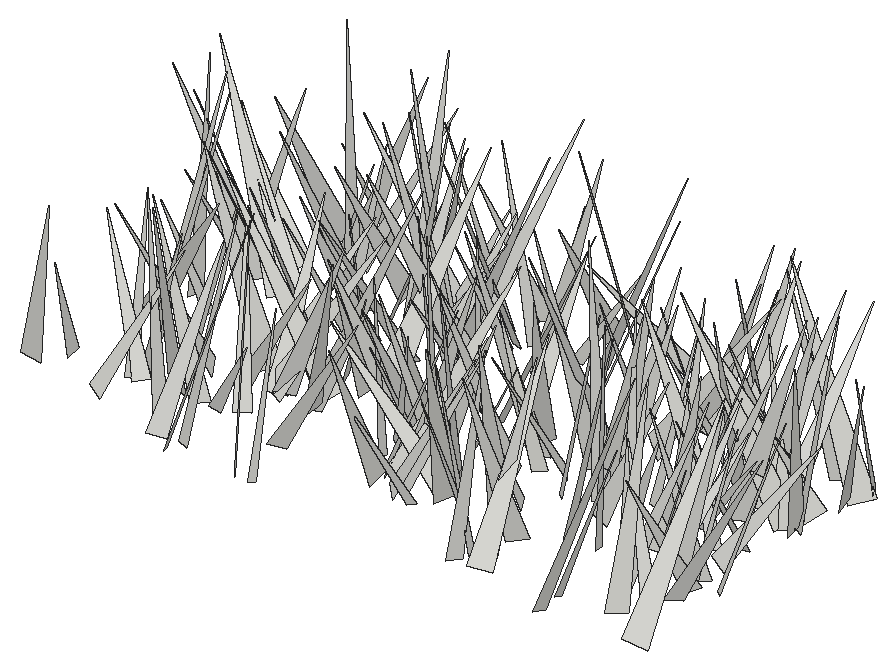
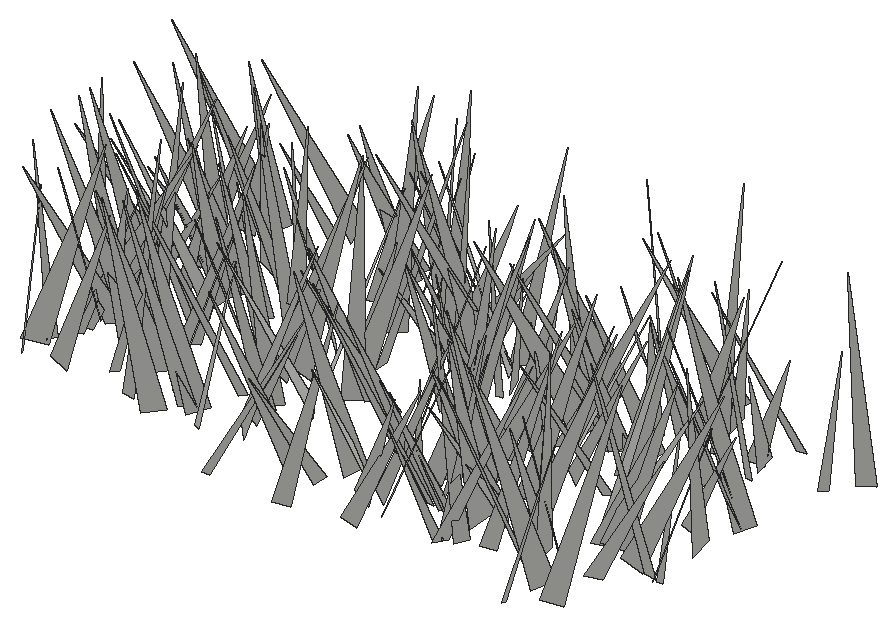
# SketchUp Ruby script. Lengths in inches.
U = 1.inch
M = Sketchup.active_model
def pt(a) = Geom::Point3d.new(a.map { |v| v * U })
def face(e, loops, mat)
  f = e.add_face(loops[0].map { |a| pt(a) })
  loops[1..].each { |l| e.add_face(l.map { |a| pt(a) }).erase! }
  f.material = f.back_material = mat if mat
  f
end
# faces: each face lists its corners as indices into pts; further lists are holes
def faces(e, pts, list, mat = nil) = list.each { |f| face(e, (f[0].is_a?(Array) ? f : [f]).map { |l| l.map { |i| pts[i] } }, mat) }
# xy, xz, yz: faces in a plane at the given z, y or x. An outline is a flat list of corners, or four numbers for a rectangle; further outlines are holes
def ring(l) = l.size == 4 ? [[l[0], l[1]], [l[2], l[1]], [l[2], l[3]], [l[0], l[3]]] : l.each_slice(2).to_a
def flat(e, list, mat, &to3) = list.each { |f| face(e, (f[0].is_a?(Array) ? f : [f]).map { |l| ring(l).map { |u, v| to3.(u, v) } }, mat) }
def xy(e, z, list, mat = nil) = flat(e, list, mat) { |x, y| [x, y, z] }
def xz(e, y, list, mat = nil) = flat(e, list, mat) { |x, z| [x, y, z] }
def yz(e, x, list, mat = nil) = flat(e, list, mat) { |y, z| [x, y, z] }
def lines(e, pts, list) = list.each { |a, b| e.add_line(pt(pts[a]), pt(pts[b])) }
# prism: a flat outline (further loops are holes) pulled along v
def prism(e, loops, v, mat = nil)
  f = face(e, loops, mat); d = Geom::Vector3d.new(v.map { |x| x * U })
  f.pushpull(f.normal.samedirection?(d) ? d.length : -d.length)
end
def box(e, o, s, mat = nil) = prism(e, [[o, [o[0] + s[0], o[1], o[2]], [o[0] + s[0], o[1] + s[1], o[2]], [o[0], o[1] + s[1], o[2]]]], [0, 0, s[2]], mat)
def at(x, y, z, deg = 0) = Geom::Transformation.translation(pt([x, y, z])) * Geom::Transformation.rotation(ORIGIN, Z_AXIS, deg.degrees)
def axes(o, x, y, z) = Geom::Transformation.new([*x, 0, *y, 0, *z, 0, *pt(o).to_a, 1])
def part(name) = M.definitions.add(name)
# library, detail: a bought-in or finely detailed component or shape, given as its bounding box
def library(name, o, s) = part(name).tap { |d| box(d.entities, o, s) }
def detail(e, o, s) = box(e.add_group.entities, o, s)
def put(e, d, t, mat = nil) = e.add_instance(d, t).tap { |i| i.material = mat if mat }
def group(e, t, mat = nil) = e.add_group.tap { |g| g.transformation = t; g.material = mat if mat }.entities
root = M.entities
c1 = part("fur_instance\#9")
p = [[0.8125,0,1.79],[0.67,-0.02,1.48],[0,-0.11,0],[0,0.11,0]]
faces(c1.entities,p,[[0,1,2,3]])
put(root,c1,axes([541.47,408.85,-21.66],[7.3603,1.92647,1.4977],[1.22652,-7.03518,3.02165],[-2.10951,2.63124,6.98247]))
put(root,c1,axes([533.68,410.5,-21.66],[-6.0255,1.4926,2.28597],[0.94971,6.33899,-1.63567],[2.5596,1.16168,5.98825]))
put(root,c1,axes([524.07,415.33,-21.66],[6.25747,-1.85529,1.59771],[-1.00282,-5.94215,-2.97253],[-2.23363,-2.52972,5.81052]))
put(root,c1,axes([516.98,410.62,-21.66],[5.31118,5.11176,2.74997],[4.78098,-5.96627,1.85658],[-3.29161,-0.41778,7.13385]))
put(root,c1,axes([548.43,409.16,-21.66],[-1.16046,8.00046,0.20395],[7.87345,1.17823,-1.41992],[1.43448,0.00519,7.95851]))
put(root,c1,axes([535.15,414.7,-21.66],[2.99002,-5.93259,1.12286],[-5.76165,-3.17812,-1.449],[-1.8055,0.31717,6.48354]))
put(root,c1,axes([531.17,414.73,-21.66],[-4.0085,-3.44331,0.94309],[-3.06456,4.04605,1.74695],[1.83147,-0.76613,4.98725]))
put(root,c1,axes([498.86,413.9375,-21.66],[1.26894,-6.32164,1.3833],[-6.3592,-0.957,1.46001],[1.19887,1.6149,6.28026]))
put(root,c1,axes([534.1,411.68,-21.66],[-5.43034,-1.89464,0.64767],[-1.9986,5.01546,-2.08529],[-0.12137,2.18018,5.36002]))
put(root,c1,axes([541.21,410.91,-21.66],[4.47299,1.54799,0.88013],[1.09405,-4.26651,1.94385],[-1.40498,1.60599,4.31572]))
put(root,c1,axes([518.46,410.37,-21.66],[1.86893,4.92203,0.04113],[4.36091,-1.67616,2.42774],[-2.28266,0.8277,4.67176]))
put(root,c1,axes([528.74,416.03,-21.66],[6.44625,-4.17663,0.34492],[-3.99481,-6.31514,-1.81045],[-1.26676,-1.33867,7.46462]))
put(root,c1,axes([527.57,414.14,-21.66],[-0.38653,-3.78857,0.47263],[-3.40937,0.1287,-1.7566],[-1.71837,0.59684,3.37891]))
put(root,c1,axes([545.21,411.5,-21.66],[-6.19625,3.45387,1.64148],[3.0912,6.3638,-1.72156],[2.25127,0.76815,6.88178]))
put(root,c1,axes([535.02,411.81,-21.66],[5.43487,-1.88004,3.06705],[-2.9758,-5.47185,1.91904],[-2.02138,3.00059,5.42123]))
put(root,c1,axes([512.02,410.2,-21.66],[6.2923,4.31715,0.79405],[3.75537,-6.01297,2.93303],[-2.27277,2.01685,7.04472]))
put(root,c1,axes([507.96,416.44,-21.66],[-1.88375,-7.99896,1.23534],[-7.80751,2.13018,1.88761],[2.13359,0.73274,7.99805]))
put(root,c1,axes([546.625,412.86,-21.66],[-1.63602,4.97918,0.62205],[4.87533,1.42244,1.43652],[-1.18757,-1.0199,5.04036]))
put(root,c1,axes([547.03,416.39,-21.66],[2.87484,-4.36178,0.57915],[-3.91954,-2.85297,-2.03053],[-1.99945,-0.67874,4.81319]))
put(root,c1,axes([512.45,411.35,-21.66],[3.92721,6.27569,0.86047],[6.07775,-4.01843,1.56873],[-1.78486,0.12492,7.23508]))
put(root,c1,axes([535.59,410.5,-21.66],[-4.59589,5.78444,0.11594],[5.4804,4.40003,-2.28044],[1.8543,1.33244,7.02721]))
put(root,c1,axes([510.55,411.1875,-21.66],[-4.56425,4.1816,0.8559],[3.58274,4.43445,-2.55936],[2.31998,1.37862,5.63629]))
put(root,c1,axes([504.38,413.08,-21.66],[2.28513,5.39499,0.34939],[5.12885,-2.04337,-1.99232],[1.70965,-1.08097,5.50984]))
put(root,c1,axes([500.49,415.91,-21.66],[4.01864,-1.00258,0.99057],[-0.63294,-3.95809,-1.43832],[-1.25928,-1.21004,3.88405]))
put(root,c1,axes([532.2,416.79,-21.66],[6.58115,-3.41587,1.26301],[-3.10443,-6.62563,-1.74311],[-1.90417,-1.00387,7.20703]))
put(root,c1,axes([516.94,414.61,-21.66],[4.74645,-3.63152,0.20608],[-3.44873,-4.38539,2.15263],[1.15614,1.82746,5.57521]))
put(root,c1,axes([509.33,413.1,-21.66],[-6.71,0.21588,0.88951],[-0.0468,6.49159,-1.92847],[0.91413,1.91692,6.43053]))
put(root,c1,axes([543.35,414.43,-21.66],[2.52048,5.79703,1.2985],[5.75928,-2.03853,-2.07834],[1.45681,-1.97061,5.96983]))
put(root,c1,axes([525.625,414.61,-21.66],[4.10268,4.53992,0.30052],[4.35228,-3.79801,-2.04106],[1.3262,-1.58032,5.76861]))
put(root,c1,axes([511.33,415.82,-21.66],[1.52564,-3.34819,0.07276],[-3.07421,-1.36842,1.48995],[1.32851,0.67846,3.36423]))
put(root,c1,axes([546.86,414.81,-21.66],[5.8068,-2.41673,0.19711],[-2.36119,-5.5195,1.88633],[0.55156,1.81463,6.0001]))
put(root,c1,axes([528.11,416.6,-21.66],[-5.02457,3.67244,0.21301],[3.24783,4.25941,3.17608],[-1.72736,-2.67378,5.35216]))
put(root,c1,axes([525.98,415.22,-21.66],[3.52755,5.08967,0.59914],[4.90233,-3.13928,-2.19532],[1.49362,-1.71683,5.79042]))
put(root,c1,axes([543.72,416.86,-21.66],[4.89387,1.35478,0.49174],[1.44124,-4.60961,-1.64362],[-0.00784,-1.71558,4.80457]))
put(root,c1,axes([528.08,417.97,-21.66],[-6.05203,-3.65216,2.90127],[-3.20675,6.70926,1.75646],[3.38709,-0.1736,6.84691]))
put(root,c1,axes([532.67,418.22,-21.66],[-3.8372,-2.33717,0.79383],[-2.01321,3.81242,1.493],[1.42812,-0.90538,4.23762]))
put(root,c1,axes([523.78,416.45,-21.66],[5.98281,3.47845,0.55141],[3.51313,-5.81778,-1.41742],[0.2481,-1.50052,6.77381]))
put(root,c1,axes([510.14,415.88,-21.66],[-1.88222,6.06948,1.49765],[6.0067,1.32242,2.18977],[-1.73238,-2.00921,5.96542]))
put(root,c1,axes([504.8,417.62,-21.66],[3.94876,4.2171,2.00571],[4.64379,-3.26946,-2.26834],[0.4919,-2.98768,5.31331]))
put(root,c1,axes([508.03,419.8,-21.66],[-6.16351,-3.9605,0.27898],[-3.73191,5.95492,2.08903],[1.35509,-1.6142,7.02213]))
put(root,c1,axes([505.7,415.86,-21.66],[-2.49681,4.68547,0.3153],[4.52882,2.308,1.56527],[-1.24213,-1.0033,5.07323]))
put(root,c1,axes([527.52,417.34,-21.66],[-0.80032,5.57612,2.90873],[5.9333,-0.30294,2.21326],[-2.08561,-3.00158,5.18026]))
put(root,c1,axes([545.11,417.35,-21.66],[0.56131,-6.10589,2.64479],[-6.41112,0.21442,1.85565],[1.78167,2.69518,5.8441]))
put(root,c1,axes([527.89,416.29,-21.66],[3.6249,6.4726,3.15784],[6.5149,-4.45394,1.65071],[-3.06961,-1.8095,7.23254]))
put(root,c1,axes([515.9,419.27,-21.66],[7.05622,-1.23215,0.51957],[-1.10047,-6.93599,-1.50315],[-0.75967,-1.39725,7.0035]))
put(root,c1,axes([546.875,417.65,-21.66],[-1.11932,5.12608,2.18052],[5.30702,0.30525,2.00664],[-1.6932,-2.43194,4.84799]))
put(root,c1,axes([525.21,417.02,-21.66],[6.77248,-2.83159,1.61361],[-3.13932,-6.6674,1.47599],[-0.87537,2.00399,7.19067]))
put(root,c1,axes([522.54,419.04,-21.66],[-1.98967,-4.65459,1.69235],[-4.24096,2.54317,2.00863],[2.55803,0.59592,4.64644]))
put(root,c1,axes([530.27,420.53,-21.66],[-7.65526,-2.65251,1.50577],[-2.23878,7.64939,2.09305],[2.07148,-1.53532,7.82675]))
put(root,c1,axes([524.98,415.8,-21.66],[0.81957,8.13408,0.73803],[7.68253,-0.51597,-2.84467],[2.77248,-0.97476,7.66439]))
put(root,c1,axes([505.1,415.71,-21.66],[-5.60466,1.1961,0.32776],[0.92969,5.05609,-2.5538],[0.82084,2.4404,5.13039]))
put(root,c1,axes([522.93,421,-21.66],[2.61621,-5.42084,0.25429],[-5.22177,-2.59146,-1.52055],[-1.47757,-0.43991,5.82391]))
put(root,c1,axes([524.6,419.02,-21.66],[-1.27388,-3.61865,0.59779],[-3.46584,0.98064,-1.44951],[-1.19998,1.0092,3.55195]))
put(root,c1,axes([542.63,419.5625,-21.66],[2.44609,-6.94499,1.47158],[-6.99231,-2.08787,1.76924],[1.22722,1.94671,7.14745]))
put(root,c1,axes([542.59,415.6875,-21.66],[1.27817,7.72916,0.81529],[7.27012,-1.48113,2.64386],[-2.74773,-0.32349,7.37453]))
put(root,c1,axes([539.55,416.85,-21.66],[-6.21182,-1.68937,2.27799],[-2.42044,6.01654,-2.13837],[1.47806,2.75267,6.07191]))
put(root,c1,axes([512.8125,416.54,-21.66],[-0.78819,5.89997,0.04998],[5.7265,0.75282,1.4401],[-1.42105,-0.23877,5.77555]))
put(root,c1,axes([510.75,418.91,-21.66],[4.20762,-3.32651,0.12048],[-3.15177,-3.91891,1.86887],[1.07075,1.53645,5.02763]))
put(root,c1,axes([537.28,416.76,-21.66],[5.41894,2.39891,1.8987],[1.67708,-5.5593,2.23748],[-2.55876,1.4367,5.48756]))
put(root,c1,axes([522.55,417.68,-21.66],[-5.22043,-0.84385,1.05571],[-1.17009,4.93002,-1.84535],[0.67639,2.01552,4.95577]))
put(root,c1,axes([528.24,417.18,-21.66],[3.83996,1.68055,0.1423],[1.49178,-3.54944,1.66307],[-0.78682,1.47206,3.84756]))
put(root,c1,axes([546.59,417.06,-21.66],[2.63197,4.07891,0.20518],[3.86496,-2.5665,1.44292],[-1.31973,0.61842,4.63495]))
put(root,c1,axes([527.16,417.83,-21.66],[3.31155,2.43431,1.59522],[1.82743,-3.61986,1.73033],[-2.2652,0.63849,3.72802]))
put(root,c1,axes([522.61,421.96,-21.66],[4.609,-3.3139,0.05026],[-3.15306,-4.41083,-1.68231],[-1.0211,-1.33793,5.42168]))
put(root,c1,axes([524.55,418.61,-21.66],[1.36791,4.73736,0.76135],[4.55305,-1.0318,-1.76027],[1.51392,-1.17738,4.60599]))
put(root,c1,axes([513.3125,419.88,-21.66],[4.4628,-4.8312,0.78242],[-4.8199,-4.15484,1.83716],[0.84924,1.80724,6.31521]))
put(root,c1,axes([542.03,418.71,-21.66],[3.72107,-3.56028,1.90501],[-4.03778,-3.30047,1.71878],[-0.03061,2.5656,4.85467]))
put(root,c1,axes([539.13,420.29,-21.66],[1.54528,-3.8993,0.59524],[-3.77652,-1.27799,1.43226],[1.13873,1.05307,3.94222]))
put(root,c1,axes([548.45,417.06,-21.66],[3.88995,3.95886,0.07672],[3.75671,-3.72392,1.68217],[-1.25122,1.12695,5.2891]))
put(root,c1,axes([537.33,419.63,-21.66],[1.43912,5.66343,2.07225],[5.60003,-0.46439,-2.61988],[2.23794,-2.47985,5.22319]))
put(root,c1,axes([544.11,417.65,-21.66],[-0.54715,4.89077,0.10405],[4.53126,0.54616,-1.84371],[1.84341,0.10915,4.56287]))
put(root,c1,axes([532.22,422.88,-21.66],[-4.33714,-4.09832,0.0827],[-3.81397,4.0787,2.10515],[1.50223,-1.4771,5.58349]))
put(root,c1,axes([515.79,421.22,-21.66],[-7.5943,2.08618,0.38061],[2.11361,7.33132,1.9887],[-0.17228,-2.01745,7.62041]))
put(root,c1,axes([501.11,422.52,-21.66],[2.01455,-7.63294,0.11302],[-6.59973,-1.68273,3.99311],[3.83642,1.11337,6.80994]))
put(root,c1,axes([510.69,421.62,-21.66],[-6.83352,3.26319,2.339],[3.80782,6.73136,1.73366],[1.27275,-2.61852,7.37155]))
put(root,c1,axes([535.85,421.7,-21.66],[-0.11111,-7.60969,2.49454],[-7.52897,0.94928,2.56048],[2.72852,2.30953,7.16685]))
put(root,c1,axes([506.48,419.22,-21.66],[5.33264,0.16428,1.51785],[-0.27785,-5.31816,1.55174],[-1.50122,1.56784,5.10452]))
put(root,c1,axes([546.19,419.82,-21.66],[1.31269,5.55847,0.82299],[4.82858,-0.68361,-3.08457],[2.8738,-1.39037,4.80678]))
put(root,c1,axes([517.03,423.04,-21.66],[4.74802,-2.11154,0.82126],[-1.70244,-4.58339,-1.94189],[-1.49491,-1.48682,4.81989]))
put(root,c1,axes([512.66,419.52,-21.66],[1.506,6.6666,0.93752],[6.04421,-0.91584,-3.19677],[2.9648,-1.51928,6.04088]))
put(root,c1,axes([543.68,418.98,-21.66],[-1.09311,5.26549,0.63584],[5.05113,1.23151,-1.51458],[1.61731,-0.28736,5.16007]))
put(root,c1,axes([515.3125,420.66,-21.66],[-5.46904,-3.01802,0.13387],[-2.92547,5.22183,-1.79189],[-0.75368,1.63119,5.98398]))
put(root,c1,axes([546.5,422.07,-21.66],[-1.81586,-4.37557,0.34615],[-4.20637,1.62778,-1.48984],[-1.25376,0.87607,4.49704]))
put(root,c1,axes([518.75,423.23,-21.66],[3.32641,-4.64571,1.36805],[-4.19977,-3.59363,-1.99171],[-2.41165,-0.14974,5.35544]))
put(root,c1,axes([544.98,420.99,-21.66],[-1.55107,4.41542,0.77186],[4.34501,1.28043,1.40671],[-1.10114,-1.16708,4.46351]))
put(root,c1,axes([523.87,422.22,-21.66],[2.085,-4.49657,0.98747],[-4.39792,-1.62495,1.88661],[1.36107,1.63764,4.58334]))
put(root,c1,axes([512.97,419.58,-21.66],[-3.56356,5.20391,0.71647],[5.00613,3.62664,-1.4419],[1.59144,0.24443,6.14008]))
put(root,c1,axes([530.97,421.98,-21.66],[-1.13244,4.66111,1.93868],[4.91983,0.57378,1.4943],[-1.13125,-2.17064,4.55801]))
put(root,c1,axes([515.75,419.28,-21.66],[7.47799,-1.52657,1.95795],[-2.25093,-6.79047,3.30259],[-1.04752,3.69369,6.88067]))
put(root,c1,axes([529.06,424.72,-21.66],[6.38115,-3.67921,0.2036],[-3.55943,-6.25987,-1.56256],[-0.95316,-1.25481,7.1982]))
put(root,c1,axes([536.32,421.18,-21.66],[0.66704,7.88186,2.68055],[8.14998,-1.16705,1.40349],[-1.69907,-2.50365,7.78452]))
put(root,c1,axes([529.87,423.34,-21.66],[-0.48012,-7.554,2.16495],[-7.6037,-0.10085,-2.03814],[-1.98335,2.21526,7.28968]))
put(root,c1,axes([533.84,420.39,-21.66],[3.8094,4.08661,1.06154],[3.80016,-3.94157,1.53675],[-1.84012,0.32005,5.37125]))
put(root,c1,axes([515.07,423.46,-21.66],[4.19489,0.81761,0.41517],[0.91291,-3.90671,-1.53042],[-0.08632,-1.58339,3.99042]))
put(root,c1,axes([542.66,422.54,-21.66],[2.65844,-2.5721,0.0216],[-2.2994,-2.3625,1.67773],[1.15278,1.21916,3.2967]))
put(root,c1,axes([523.16,426.28,-21.66],[-4.76497,-3.93422,0.44703],[-3.2824,4.31602,2.99679],[2.21445,-2.06803,5.40391]))
put(root,c1,axes([542.42,420.28,-21.66],[-6.84761,2.51212,1.52779],[1.98246,6.80446,-2.30302],[2.17135,1.70976,6.92074]))
put(root,c1,axes([534.45,425.11,-21.66],[-1.86183,-7.54983,1.10161],[-7.50699,1.61006,-1.65309],[-1.3633,1.44488,7.59827]))
put(root,c1,axes([503.11,420.83,-21.66],[5.00071,5.94343,0.88428],[5.7504,-5.06729,1.53914],[-1.74336,0.3341,7.61331]))
put(root,c1,axes([533.54,424.19,-21.66],[-0.98581,-7.65367,2.64082],[-7.9173,0.35473,-1.92744],[-1.69382,2.79641,7.47232]))
put(root,c1,axes([513.05,424,-21.66],[-3.40667,-4.88664,0.79026],[-4.79108,3.01371,-2.01797],[-1.2447,1.77411,5.60468]))
put(root,c1,axes([507.74,427.43,-21.66],[-4.53794,-6.8341,0.16977],[-6.57814,4.42074,2.12406],[1.86058,-1.03861,7.92377]))
put(root,c1,axes([547.21,425.95,-21.66],[7.02659,-0.33713,1.59],[0.09653,-6.95626,-1.90152],[-1.62247,-1.87389,6.7728]))
put(root,c1,axes([542.24,423.5,-21.66],[3.65176,6.04586,1.11201],[6.02251,-3.25936,-2.05677],[1.23222,-1.98709,6.75703]))
put(root,c1,axes([503.86,424.64,-21.66],[-0.24742,-3.68689,1.2628],[-3.55064,-0.30834,-1.59591],[-1.60648,1.24932,3.33279]))
put(root,c1,axes([542.32,421.5,-21.66],[7.12213,3.78972,1.00867],[3.4176,-7.02352,2.25704],[-1.92338,1.55314,7.74548]))
put(root,c1,axes([546.34,426.1,-21.66],[-7.92246,2.32052,1.49756],[2.68865,7.5204,2.57051],[0.63138,-2.90715,7.84491]))
put(root,c1,axes([542.16,427.15,-21.66],[-1.3783,-7.92591,0.91068],[-7.76861,1.54372,1.6777],[1.81604,0.58822,7.86798]))
put(root,c1,axes([512.99,426.9,-21.66],[-4.86193,-2.9811,0.43497],[-2.74592,4.72474,1.68858],[1.2394,-1.22654,5.44739]))
put(root,c1,axes([540.83,425.5,-21.66],[-5.87282,3.13064,1.60123],[3.47052,5.66214,1.65846],[0.56601,-2.23474,6.44519]))
put(root,c1,axes([513.48,427.7,-21.66],[3.27903,-5.74844,0.73311],[-5.41958,-3.34021,-1.9507],[-2.05188,-0.36394,6.32387]))
put(root,c1,axes([534.95,425.02,-21.66],[-0.35143,6.05342,2.99786],[6.31844,1.35633,-1.99808],[2.38924,-2.69649,5.72495]))
put(root,c1,axes([543.76,424.61,-21.66],[6.10397,-4.61293,1.81963],[-4.95361,-5.80478,1.9013],[-0.22786,2.62185,7.41098]))
put(root,c1,axes([502.4,421.9,-21.66],[3.79972,6.90357,0.39781],[6.61789,-3.76205,2.07507],[-2.00527,0.66563,7.60206]))
put(root,c1,axes([516.72,427.65,-21.66],[0.00181,-5.98408,0.19016],[-5.68264,-0.06159,-1.88392],[-1.88493,0.17992,5.67979]))
put(root,c1,axes([538.9,422.9,-21.66],[2.7978,5.22834,0.27095],[4.99402,-2.75746,1.64099],[-1.57121,0.54549,5.69828]))
put(root,c1,axes([547.18,427.78,-21.66],[-6.27712,3.42033,1.55819],[3.73626,5.34865,3.31076],[-0.40863,-3.63622,6.33559]))
put(root,c1,axes([510.05,424.32,-21.66],[1.05381,5.0713,0.10966],[4.76326,-0.95083,-1.80217],[1.74396,-0.4674,4.856]))
put(root,c1,axes([527.99,423.87,-21.66],[-2.51338,5.74575,1.01303],[5.46798,2.70448,-1.77311],[2.03497,-0.17044,6.01555]))
put(root,c1,axes([520.58,424.95,-21.66],[-5.03149,-1.83162,1.20846],[-2.18082,4.50919,-2.24552],[0.24343,2.5384,4.86091]))
put(root,c1,axes([519.12,429.8,-21.66],[-7.73279,0.49202,2.83462],[1.75633,7.24586,3.53356],[2.27869,-3.91518,6.89581]))
put(root,c1,axes([546.6875,428.57,-21.66],[-4.22388,-0.55824,1.0602],[-0.01996,3.91714,1.98304],[1.19803,-1.90295,3.77099]))
put(root,c1,axes([543.84,427.08,-21.66],[4.37755,-6.1842,1.75356],[-6.40379,-4.01166,1.83857],[0.55746,2.47882,7.3503]))
put(root,c1,axes([546.74,425.59,-21.66],[-0.83276,5.81039,0.96307],[5.68734,0.54058,1.65638],[-1.53047,-1.15272,5.63121]))
put(root,c1,axes([532.32,428.17,-21.66],[1.87666,-6.19619,1.68038],[-6.32701,-1.4881,1.57887],[1.08876,2.03251,6.27868]))
put(root,c1,axes([517.32,424.74,-21.66],[-1.94232,7.80928,1.11049],[7.41359,2.19794,-2.48968],[2.69386,-0.41817,7.65238]))
put(root,c1,axes([501.77,425.93,-21.66],[-7.13651,-0.0123,2.39844],[-0.61978,7.28244,-1.80677],[2.31701,1.91008,6.90402]))
put(root,c1,axes([525.49,425.04,-21.66],[6.20269,2.14266,0.41588],[1.88774,-5.89525,2.21806],[-1.09562,1.97291,6.17613]))
put(root,c1,axes([538.27,430.26,-21.66],[-4.62318,-3.47557,0.41553],[-3.19467,4.47097,1.85217],[1.4305,-1.24775,5.47931]))
put(root,c1,axes([544.24,426.39,-21.66],[-0.17327,7.80384,1.95788],[7.72096,0.71202,-2.15474],[2.26272,-1.83203,7.50246]))
put(root,c1,axes([519.29,428.62,-21.66],[-0.93338,-7.69941,2.7531],[-7.87622,0.10215,-2.38461],[-2.19672,2.90522,7.38009]))
put(root,c1,axes([501.56,430.66,-21.66],[-3.93384,-2.91751,0.42121],[-2.51987,3.69278,2.04402],[1.52955,-1.41982,4.45073]))
put(root,c1,axes([547.47,425.83,-21.66],[3.93388,5.26717,1.14139],[4.90502,-4.08461,1.94372],[-2.23307,0.30691,6.28017]))
put(root,c1,axes([542.2,430.87,-21.66],[-5.45284,-1.57742,1.94379],[-0.6971,5.43147,2.45217],[2.40429,-2.00271,5.11943]))
put(root,c1,axes([506.74,428.4,-21.66],[-5.49378,-4.48735,0.1731],[-4.21573,5.05933,-2.64174],[-1.54724,2.14821,6.58325]))
put(root,c1,axes([547.57,430.06,-21.66],[5.98567,0.36805,0.66862],[0.55714,-5.71998,-1.83907],[-0.52163,-1.88604,5.70802]))
put(root,c1,axes([534.47,428.38,-21.66],[4.68753,6.76488,0.69054],[6.04009,-3.75687,-4.19721],[3.12373,-2.88717,7.07954]))
put(root,c1,axes([510.81,430.69,-21.66],[0.32689,-6.93131,1.01824],[-6.72809,-0.59471,-1.88835],[-1.95261,0.88881,6.67713]))
put(root,c1,axes([501.14,430.625,-21.66],[-2.16154,-4.08693,0.6496],[-3.73051,2.24163,1.68984],[1.79115,-0.26331,4.30345]))
put(root,c1,axes([510.66,430.44,-21.66],[-2.98653,-2.99705,1.42564],[-2.58075,3.30304,1.53746],[2.08674,-0.20437,3.94181]))
put(root,c1,axes([532.27,428.91,-21.66],[0.67083,5.9533,2.27987],[6.17356,-0.03505,-1.72498],[1.58958,-2.37626,5.73727]))
put(root,c1,axes([545.71,426.2,-21.66],[-2.00066,7.03095,0.19663],[6.73059,1.97306,-2.06922],[2.04255,0.38513,7.01108]))
put(root,c1,axes([503.68,430.08,-21.66],[-2.36054,6.29762,2.85628],[6.53149,1.03928,3.10644],[-2.27111,-3.55673,5.96508]))
put(root,c1,axes([521.4,428.15,-21.66],[-4.31752,-0.25034,0.73123],[-0.52227,4.00392,-1.71296],[0.56974,1.77322,3.97108]))
put(root,c1,axes([539.76,432.64,-21.66],[-3.16207,-7.07316,1.24758],[-6.76016,3.39142,2.09364],[2.42619,0.2311,7.45956]))
put(root,c1,axes([530.11,427.16,-21.66],[5.9455,4.2001,0.21568],[4.05072,-5.81939,1.66213],[-1.13095,1.23699,7.08711]))
put(root,c1,axes([515.97,427.88,-21.66],[6.62272,2.03005,2.53711],[1.31072,-6.93962,2.13125],[-2.97322,1.46257,6.59085]))
put(root,c1,axes([520.82,431.85,-21.66],[-4.32918,-1.79601,0.73607],[-1.48596,4.22424,1.56749],[1.24875,-1.19977,4.41706]))
put(root,c1,axes([506.58,429.26,-21.66],[-3.94655,4.7323,0.06828],[4.56087,3.77904,1.70056],[-1.26405,-1.13963,5.92267]))
put(root,c1,axes([505.78,429.01,-21.66],[-4.22364,6.9226,0.63988],[6.72709,3.88063,2.42031],[-1.75445,-1.78585,7.73974]))
put(root,c1,axes([511.64,433.71,-21.66],[6.11084,-2.63091,1.80363],[-1.49433,-5.80472,-3.40432],[-2.81811,-2.62692,5.71618]))
put(root,c1,axes([532.14,430.39,-21.66],[-1.49858,-3.44059,1.04989],[-3.40031,0.98374,-1.62968],[-1.17382,1.54281,3.38047]))
put(root,c1,axes([501.99,430.41,-21.66],[3.4737,5.90005,1.74495],[6.11319,-3.08303,-1.74525],[0.69596,-2.36778,6.62052]))
put(root,c1,axes([548,432.37,-21.66],[-3.52584,-3.38703,1.52089],[-2.9555,3.82986,1.67745],[2.24724,-0.27722,4.59235]))
put(root,c1,axes([548.17,430.98,-21.66],[-5.06971,5.94983,1.91077],[6.22333,4.58369,2.23904],[-0.56711,-2.88838,7.48926]))
put(root,c1,axes([535.36,431.5,-21.66],[5.33015,-4.46349,0.382],[-4.4244,-5.15196,1.5366],[0.7024,1.41905,6.78027]))
put(root,c1,axes([534.23,433.06,-21.66],[-3.15103,-4.03715,0.66571],[-3.75697,3.18756,1.54769],[1.62077,-0.46003,4.88182]))
put(root,c1,axes([540,429.12,-21.66],[-2.57926,6.41675,1.59968],[6.21683,2.93816,-1.76197],[2.25493,-0.76079,6.68751]))
put(root,c1,axes([515.35,428.92,-21.66],[-5.11664,3.91829,0.85035],[3.38571,4.96082,-2.48663],[2.14782,1.51438,5.94556]))
put(root,c1,axes([517.5,430.5,-21.66],[-6.96753,-1.64469,0.65915],[-1.76863,6.61713,-2.18437],[0.10697,2.27915,6.81763]))
put(root,c1,axes([532.0625,431.45,-21.66],[-6.33694,-5.31771,1.42218],[-5.44687,5.74429,-2.79146],[-0.79519,3.03026,7.78734]))
put(root,c1,axes([520.47,432.95,-21.66],[-3.35511,-5.27651,0.83113],[-5.27558,3.11951,-1.49198],[-0.83701,1.48869,6.07225]))
put(root,c1,axes([536.2,431.48,-21.66],[0.74046,6.81709,2.01452],[6.9144,-0.22063,-1.79488],[1.64984,-2.13492,6.61811]))
put(root,c1,axes([513.3125,434.11,-21.66],[7.4678,0.08394,0.57516],[0.2355,-7.21321,-2.00499],[-0.53141,-2.01703,7.1941]))
put(root,c1,axes([515.43,432.6875,-21.66],[2.92691,3.10527,0.26779],[2.82947,-2.4932,-2.01476],[1.3071,-1.55642,3.76168]))
put(root,c1,axes([504.56,432.63,-21.66],[-4.43376,3.47486,0.22998],[3.34427,4.14468,1.85019],[-0.97128,-1.59146,5.32068]))
put(root,c1,axes([545.39,432.16,-21.66],[-0.37721,6.24874,2.25952],[6.16262,-0.51732,2.45945],[-2.4848,-2.23161,5.75674]))
put(root,c1,axes([516.48,431.7,-21.66],[0.2906,4.64928,0.9365],[4.41539,0.07727,-1.75374],[1.73123,-0.9775,4.31562]))
put(root,c1,axes([506.51,433.03,-21.66],[3.8282,2.91024,0.83789],[3.01788,-3.55309,-1.44728],[0.25298,-1.65308,4.58585]))
put(root,c1,axes([509.3125,431.22,-21.66],[4.39596,-0.31282,2.17467],[-1.10489,-4.51925,1.5834],[-1.89902,1.90528,4.11281]))
put(root,c1,axes([517.9,431.08,-21.66],[6.72656,-0.08852,1.07497],[-0.40385,-6.50233,1.99163],[-1.00015,2.03024,6.42556]))
put(root,c1,axes([523.47,431.46,-21.66],[6.60662,-2.19065,2.41659],[-2.83754,-6.55209,1.81792],[-1.6085,2.56075,6.71874]))
put(root,c1,axes([512.93,430.23,-21.66],[4.98815,3.01806,0.37753],[2.59556,-4.60182,2.49383],[-1.58564,1.9615,5.26983]))
put(root,c1,axes([515.75,432.36,-21.66],[-7.81157,-0.92448,1.21309],[-1.13809,7.74743,-1.42443],[1.01538,1.5715,7.73604]))
put(root,c1,axes([537.4,433.18,-21.66],[3.87683,-5.48097,2.21285],[-5.90731,-3.50163,1.67625],[0.20355,2.76859,6.50085]))
put(root,c1,axes([523.26,430.89,-21.66],[3.56764,3.88458,0.34534],[3.52617,-3.41301,1.96335],[-1.66594,1.09483,4.89523]))
put(root,c1,axes([514.37,434.84,-21.66],[-6.85321,0.30824,0.48855],[0.41589,6.6696,1.62593],[0.40091,-1.64973,6.66467]))
put(root,c1,axes([504.55,436.58,-21.66],[4.75153,-4.99406,0.9078],[-4.47168,-4.70683,-2.48828],[-2.40183,-1.11663,6.42854]))
put(root,c1,axes([518.02,431.64,-21.66],[3.14457,7.68443,0.45621],[7.56933,-2.99688,-1.69436],[1.40136,-1.05601,8.12822]))
put(root,c1,axes([508.48,432.46,-21.66],[-8.04005,-0.21045,2.18635],[-0.63833,8.16213,-1.56173],[2.10165,1.67397,7.88972]))
put(root,c1,axes([530.3,437.08,-21.66],[-5.57045,-1.42182,0.3414],[-1.0257,4.7578,3.07884],[1.04215,-2.91715,4.85512]))
put(root,c1,axes([524.47,437.26,-21.66],[5.34512,-3.23236,0.64666],[-2.65449,-4.95104,-2.80671],[-1.95449,-2.11559,5.5804]))
put(root,c1,axes([519.36,433.75,-21.66],[-6.43064,-2.17008,0.24743],[-2.17262,6.27662,-1.4168],[-0.22404,1.42068,6.6374]))
put(root,c1,axes([513.97,431.4,-21.66],[-7.73799,2.57835,1.8542],[1.9672,7.72518,-2.53263],[2.4932,1.90688,7.75308]))
put(root,c1,axes([524.48,433.55,-21.66],[3.53802,-1.77872,0.68161],[-1.86523,-2.94336,2.00089],[0.38644,2.07817,3.41729]))
put(root,c1,axes([514.57,434.85,-21.66],[0.74077,3.76285,1.03817],[3.63302,-0.27816,-1.5841],[1.42759,-1.24465,3.49262]))
put(root,c1,axes([520,436.46,-21.66],[0.21984,-5.04241,1.33274],[-4.72838,-0.75562,-2.0789],[-2.20101,1.11963,4.59917]))
put(root,c1,axes([526.34,433.6,-21.66],[6.82155,0.82248,0.97272],[0.53436,-6.65794,1.88216],[-1.15634,1.77527,6.60814]))
put(root,c1,axes([521.23,433.67,-21.66],[0.1109,6.16383,0.84068],[5.38265,-0.51661,3.07768],[-3.11876,-0.67243,5.34163]))
put(root,c1,axes([506.21,435.26,-21.66],[6.24865,-3.61776,1.18124],[-3.80474,-5.99015,1.78079],[-0.08657,2.13519,6.99733]))
put(root,c1,axes([507.19,435.07,-21.66],[4.17015,5.48726,0.52169],[5.30168,-3.81404,-2.26221],[1.50809,-1.76505,6.51019]))
put(root,c1,axes([506.85,438.23,-21.66],[-4.18199,-2.55213,0.91155],[-1.98836,4.02848,2.15666],[1.84139,-1.44616,4.39901]))
